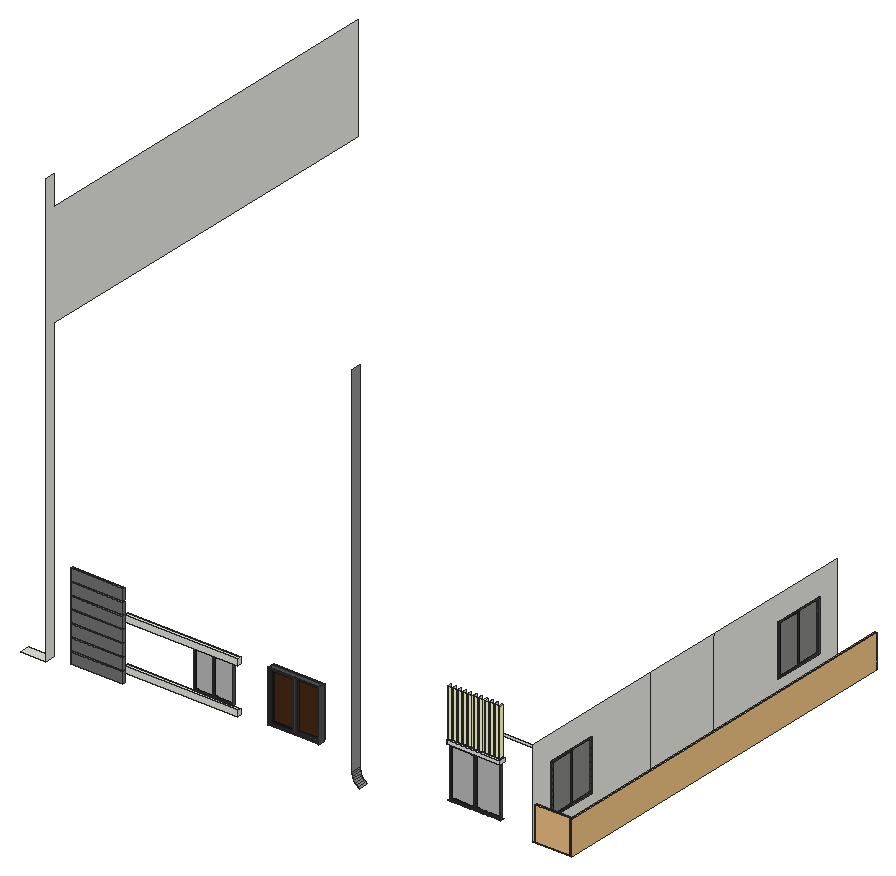
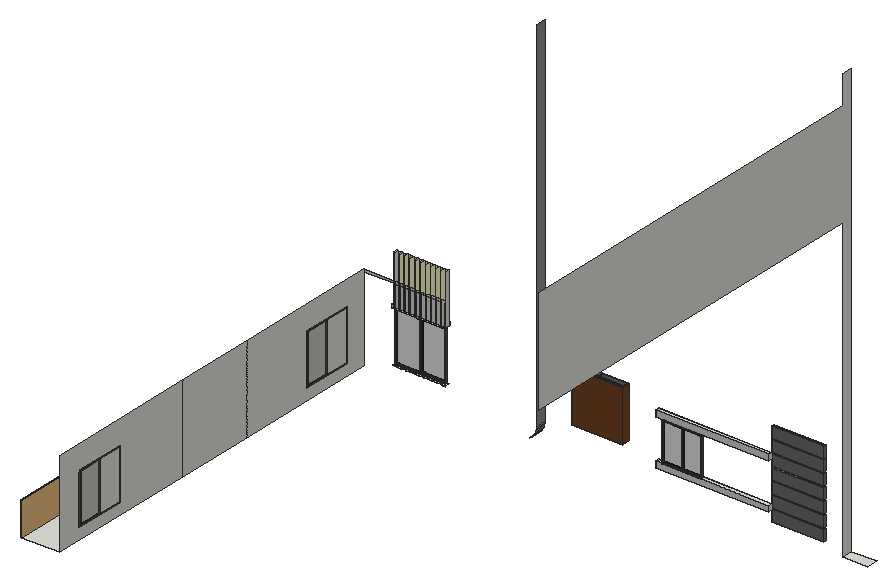
# SketchUp Ruby script. Lengths in inches.
U = 1.inch
M = Sketchup.active_model
def pt(a) = Geom::Point3d.new(a.map { |v| v * U })
def face(e, loops, mat)
  f = e.add_face(loops[0].map { |a| pt(a) })
  loops[1..].each { |l| e.add_face(l.map { |a| pt(a) }).erase! }
  f.material = f.back_material = mat if mat
  f
end
# faces: each face lists its corners as indices into pts; further lists are holes
def faces(e, pts, list, mat = nil) = list.each { |f| face(e, (f[0].is_a?(Array) ? f : [f]).map { |l| l.map { |i| pts[i] } }, mat) }
# xy, xz, yz: faces in a plane at the given z, y or x. An outline is a flat list of corners, or four numbers for a rectangle; further outlines are holes
def ring(l) = l.size == 4 ? [[l[0], l[1]], [l[2], l[1]], [l[2], l[3]], [l[0], l[3]]] : l.each_slice(2).to_a
def flat(e, list, mat, &to3) = list.each { |f| face(e, (f[0].is_a?(Array) ? f : [f]).map { |l| ring(l).map { |u, v| to3.(u, v) } }, mat) }
def xy(e, z, list, mat = nil) = flat(e, list, mat) { |x, y| [x, y, z] }
def xz(e, y, list, mat = nil) = flat(e, list, mat) { |x, z| [x, y, z] }
def yz(e, x, list, mat = nil) = flat(e, list, mat) { |y, z| [x, y, z] }
def lines(e, pts, list) = list.each { |a, b| e.add_line(pt(pts[a]), pt(pts[b])) }
# prism: a flat outline (further loops are holes) pulled along v
def prism(e, loops, v, mat = nil)
  f = face(e, loops, mat); d = Geom::Vector3d.new(v.map { |x| x * U })
  f.pushpull(f.normal.samedirection?(d) ? d.length : -d.length)
end
def box(e, o, s, mat = nil) = prism(e, [[o, [o[0] + s[0], o[1], o[2]], [o[0] + s[0], o[1] + s[1], o[2]], [o[0], o[1] + s[1], o[2]]]], [0, 0, s[2]], mat)
def at(x, y, z, deg = 0) = Geom::Transformation.translation(pt([x, y, z])) * Geom::Transformation.rotation(ORIGIN, Z_AXIS, deg.degrees)
def axes(o, x, y, z) = Geom::Transformation.new([*x, 0, *y, 0, *z, 0, *pt(o).to_a, 1])
def part(name) = M.definitions.add(name)
# library, detail: a bought-in or finely detailed component or shape, given as its bounding box
def library(name, o, s) = part(name).tap { |d| box(d.entities, o, s) }
def detail(e, o, s) = box(e.add_group.entities, o, s)
def put(e, d, t, mat = nil) = e.add_instance(d, t).tap { |i| i.material = mat if mat }
def group(e, t, mat = nil) = e.add_group.tap { |g| g.transformation = t; g.material = mat if mat }.entities
root = M.entities
M.materials.add("Glass_Tinted_Gray").color = [0, 0, 0]
M.materials["Glass_Tinted_Gray"].alpha = 0.125
M.materials.add("[0135_DarkGray]").color = [81, 81, 81]
M.materials.add("[Color E01]").color = [255, 255, 204]
M.materials.add("[Color M04]").color = [142, 142, 142]
M.materials.add("[Color M05]").color = [114, 114, 114]
M.materials.add("[Mirror 02]").color = [229, 229, 229]
M.materials.add("[Terrazzo Light Blue]").color = [196, 214, 227]
M.materials.add("[Wood Veneer 01]").color = [120, 70, 37]
c1 = library("Wagner Glass Railing",[9.08,102.375,1.53],[2.51,145.5,42.05])
c2 = part("Group\#9")
box(c2.entities,[0,-2.75,0],[65.625,2.75,13.9375])
c3 = part("PENTEK_RP Fineline 50S_Sliding_DoorCase_E1")
box(c3.entities,[0,0,0],[1.51,3.66,99.27],"[0135_DarkGray]")
c4 = part("PENTEK_RP Fineline 50S_SlidingDooe_Case_E2")
box(c4.entities,[0,0,0],[96.25,3.66,1.51],"[0135_DarkGray]")
c5 = part("pentek_RP Fineline 50S_SlidingDoor_Case")
put(c5.entities,c3,at(97.76,0,0))
put(c5.entities,c4,at(1.51,0,0))
put(c5.entities,c3,at(0,0,0))
put(c5.entities,c4,at(1.51,0,97.76))
c6 = part("PENTEK_RP Fineline 50S_SlidingDoor_GlazingBead_2")
box(c6.entities,[0,0,0],[0.56,0.59,94.39],"[0135_DarkGray]")
c7 = part("PENTEK_RP Fineline 50S_SlidingDoor_Glass")
box(c7.entities,[0,0,0],[46.58,0.16,94.39],"Glass_Tinted_Gray")
c8 = part("PENTEK_RP Fineline 50S_SlidingDoor_GlazingBead")
box(c8.entities,[0,0,0],[45.47,0.59,0.56],"[0135_DarkGray]")
c9 = part("PENTEK_RP Fineline 50S_SlidingDoor_Leaf_E1")
xy(c9.entities,0,[[0,0,0.93,1.97],[0.93,1.57,1.49,1.97]],"[0135_DarkGray]")
xy(c9.entities,96.25,[[0,0,0.93,0,0.93,1.57,1.49,1.57,1.49,1.97,0,1.97]],"[0135_DarkGray]")
xz(c9.entities,0,[[0,0,0.93,96.25]],"[0135_DarkGray]")
xz(c9.entities,1.57,[[0.93,0,1.49,95.32],[0.93,95.32,1.49,96.25]],"[0135_DarkGray]")
xz(c9.entities,1.97,[[0,0,1.49,96.25]],"[0135_DarkGray]")
yz(c9.entities,0,[[0,0,1.97,96.25]],"[0135_DarkGray]")
yz(c9.entities,0.93,[[0,0,1.57,0.93],[0,0.93,1.57,95.32],[0,95.32,1.57,96.25]],"[0135_DarkGray]")
yz(c9.entities,1.49,[[1.57,0,1.97,95.32],[1.57,95.32,1.97,96.25]],"[0135_DarkGray]")
c10 = part("PENTEK_RP Fineline 50S_SlidingDoor_Leaf_E2")
xy(c10.entities,0,[[0,0,0,1.57,0.56,1.57,0.56,1.97,46.02,1.97,46.02,1.57,46.58,1.57,46.58,0]],"[0135_DarkGray]")
xy(c10.entities,0.93,[[0,0,46.58,1.57]],"[0135_DarkGray]")
xy(c10.entities,1.49,[[0.56,1.57,46.02,1.97]],"[0135_DarkGray]")
xz(c10.entities,0,[[0,0,46.58,0.93]],"[0135_DarkGray]")
xz(c10.entities,1.57,[[0,0,0.56,0.93],[46.02,0,46.58,0.93],[0.56,0.93,46.02,1.49]],"[0135_DarkGray]")
xz(c10.entities,1.97,[[0.56,0,46.02,1.49]],"[0135_DarkGray]")
yz(c10.entities,0,[[0,0,1.57,0.93]],"[0135_DarkGray]")
yz(c10.entities,0.56,[[1.57,0,1.97,0.93],[1.57,0.93,1.97,1.49]],"[0135_DarkGray]")
yz(c10.entities,46.02,[[1.57,0,1.97,0.93],[1.57,0.93,1.97,1.49]],"[0135_DarkGray]")
yz(c10.entities,46.58,[[0,0,1.57,0.93]],"[0135_DarkGray]")
c11 = part("PENTEK_RP Fineline S_SlidingDoor_Leaf1")
put(c11.entities,c6,at(0.93,0,0.93))
put(c11.entities,c6,at(46.96,0,0.93))
put(c11.entities,c7,at(1.49,1.42,0.93))
put(c11.entities,c8,at(1.49,0,0.93))
put(c11.entities,c7,at(1.49,0.59,0.93),"[Terrazzo Light Blue]")
put(c11.entities,c9,at(0,0,0))
put(c11.entities,c9,axes([48.44,0,0],[-1,0,0],[0,1,0],[0,0,1]))
put(c11.entities,c10,axes([0.93,0,96.25],[1,0,0],[0,1,0],[0,0,-1]))
put(c11.entities,c10,at(0.93,0,0))
put(c11.entities,c8,at(1.49,0,94.77))
c12 = part("PENTEK_RP Fineline 50S_SlidingDoor_Leaf2")
put(c12.entities,c7,at(1.49,1.42,0.93))
put(c12.entities,c8,at(1.49,0,94.77))
put(c12.entities,c6,at(46.96,0,0.93))
put(c12.entities,c7,at(1.49,0.59,0.93),"[Mirror 02]")
put(c12.entities,c6,at(0.93,0,0.93))
put(c12.entities,c9,at(0,0,0))
put(c12.entities,c9,axes([48.44,0,0],[-1,0,0],[0,1,0],[0,0,1]))
put(c12.entities,c8,at(1.49,0,0.93))
put(c12.entities,c10,axes([0.93,0,96.25],[1,0,0],[0,1,0],[0,0,-1]))
put(c12.entities,c10,at(0.93,0,0))
c13 = part("PENTEK - Slimmest Steel Sliding Door / Window\#1")
put(c13.entities,c5,at(0,-1.88,-0.09))
put(c13.entities,c11,at(1.51,-2.27,1.42))
put(c13.entities,c12,at(49.32,-0.3,1.42))
c14 = part("Group\#10")
box(c14.entities,[-76.71,-4.875,-2.4375],[142.83,4.875,7.6875])
xy(root,7.25,[[7.375,49.27,39.25,62.39]])
xy(root,10.57,[[643.25,62.39,690.1875,542.39]])
xy(root,23.9,[[540.26,57.14,545.19,62.39],[545.88,57.14,550.82,62.39],[551.38,57.14,556.32,62.39],[557.13,57.14,562.07,62.39],[562.82,57.14,567.76,62.39],
  [568.44,57.14,573.38,62.39],[574.07,57.14,579.01,62.39],[579.51,57.14,584.44,62.39],[585.32,57.14,590.26,62.39],[590.94,57.14,595.88,62.39],
  [596.88,57.14,601.82,62.39],[602.25,57.14,607.1875,62.39]])
xy(root,34.3125,[[318.6,50.27,382.47,59.77]],"[Wood Veneer 01]")
xy(root,88.25,[[540.59,54.54,608.4,62.39]])
xy(root,90.0625,[[540.39,57.14,540.59,62.39],[540.59,57.14,545.76,62.39],[546.71,57.14,552.08,62.39],[553.03,57.14,558.4,62.39],[559.28,57.14,564.65,62.39],
  [565.65,57.14,571.03,62.39],[572.84,57.14,578.21,62.39],[579.65,57.14,585.03,62.39],[586.71,57.14,592.09,62.39],[592.73,57.14,598.11,62.39],
  [599.11,57.14,606.05,62.39]])
xy(root,93.1875,[[540.59,54.54,608.4,54.54,608.4,62.39,606.05,62.39,606.05,57.14,599.11,57.14,599.11,62.39,598.11,62.39,598.11,57.14,592.73,57.14,592.73,62.39,592.09,62.39,592.09,57.14,586.71,57.14,586.71,62.39,585.03,62.39,585.03,57.14,579.65,57.14,579.65,62.39,578.21,62.39,578.21,57.14,572.84,57.14,572.84,62.39,571.03,62.39,571.03,57.14,565.65,57.14,565.65,62.39,564.65,62.39,564.65,57.14,559.28,57.14,559.28,62.39,558.4,62.39,558.4,57.14,553.03,57.14,553.03,62.39,552.08,62.39,552.08,57.14,546.71,57.14,546.71,62.39,545.76,62.39,545.76,57.14,540.59,57.14]])
xy(root,98.1875,[[318.6,50.27,382.47,59.77]],"[Wood Veneer 01]")
xz(root,54.54,[[540.59,88.25,608.4,93.1875]])
xz(root,57.14,[[540.59,90.0625,545.76,93.1875],[546.71,90.0625,546.91,93.1875],[546.91,90.0625,552.08,93.1875],[553.03,90.0625,553.23,93.1875],[553.23,90.0625,558.4,93.1875],
  [559.28,90.0625,559.48,93.1875],[559.48,90.0625,564.65,93.1875],[565.65,90.0625,565.85,93.1875],[565.85,90.0625,571.03,93.1875],[572.84,90.0625,573.04,93.1875],
  [573.04,90.0625,578.21,93.1875],[579.65,90.0625,579.85,93.1875],[579.85,90.0625,585.03,93.1875],[586.71,90.0625,586.92,93.1875],[586.92,90.0625,592.09,93.1875],
  [592.73,90.0625,592.9375,93.1875],[592.9375,90.0625,598.11,93.1875],[599.11,90.0625,599.3125,93.1875],[604.48,90.0625,606.05,93.1875]])
xz(root,57.14,[[540.39,90.0625,540.59,90.0625,540.59,93.1875,545.76,93.1875,545.76,152.27,540.39,152.27],[599.3125,90.0625,604.48,90.0625,604.48,93.1875,606.05,93.1875,606.05,152.27,604.48,152.27,604.48,93.1875,599.3125,93.1875],[546.71,93.1875,552.08,152.27],[553.03,93.1875,558.4,152.27],[559.28,93.1875,564.65,152.27],
  [565.65,93.1875,571.03,152.27],[572.84,93.1875,578.21,152.27],[579.65,93.1875,585.03,152.27],[586.71,93.1875,592.09,152.27],[592.73,93.1875,598.11,152.27],
  [599.11,93.1875,604.48,152.27]],"[Color E01]")
xz(root,59.77,[[318.6,34.3125,382.47,98.1875]],"[Wood Veneer 01]")
xz(root,62.39,[[540.39,90.0625,541.21,116.82],[541.21,90.0625,545.76,90.0625,545.76,120,540.39,120,540.39,116.82,541.21,116.82],[546.71,90.0625,552.08,116.82],[553.03,90.0625,558.4,116.82],[559.28,90.0625,564.65,116.82],
  [565.65,90.0625,571.03,116.82],[572.84,90.0625,578.21,116.82],[579.65,90.0625,585.03,116.82],[586.71,90.0625,592.09,116.82],[592.73,90.0625,598.11,116.82],
  [599.11,90.0625,604.48,116.82],[604.48,90.0625,606.05,116.82],[545.76,93.1875,546.27,93.1875,546.27,116.82,546.71,116.82,546.71,120,545.76,120],[546.27,93.1875,546.71,116.82],[552.08,93.1875,553.03,116.82],
  [558.4,93.1875,559.28,116.82],[564.65,93.1875,565.65,116.82],[571.03,93.1875,572.84,116.82],[578.21,93.1875,579.65,116.82],[585.03,93.1875,586.71,116.82],
  [592.09,93.1875,592.73,116.82],[598.11,93.1875,599.11,116.82],[539.4375,116.82,540.39,120],[546.71,116.82,552.08,120],[552.08,116.82,553.03,120],
  [553.03,116.82,558.4,120],[558.4,116.82,559.28,120],[559.28,116.82,564.65,116.82,564.65,119.69,561.41,119.69,561.41,120,559.28,120],[564.65,116.82,565.65,119.69],[565.65,116.82,571.03,119.69],
  [571.03,116.82,572.84,119.69],[572.84,116.82,578.21,119.69],[578.21,116.82,579.65,119.69],[579.65,116.82,585.03,119.69],[585.03,116.82,586.71,119.69],
  [586.71,116.82,592.09,119.69],[592.09,116.82,592.73,119.69],[592.73,116.82,598.11,119.69],[598.11,116.82,599.11,119.69],[599.11,116.82,604.48,119.69],
  [604.48,116.82,606.05,119.69],[606.05,116.82,643.25,119.69]])
yz(root,39.25,[[49.27,7.25,49.27,552.6875,62.39,552.6875,62.39,516,542.39,516,542.39,384,62.39,384,62.39,7.25]])
yz(root,318.6,[[50.27,34.3125,59.77,98.1875]],"[Wood Veneer 01]")
yz(root,382.47,[[50.27,34.3125,59.77,98.1875]],"[Wood Veneer 01]")
yz(root,425.1875,[[50.27,18.35,62.39,472.24]],"[Color M04]")
yz(root,540.39,[[57.14,90.0625,62.39,152.27]])
yz(root,540.59,[[54.54,88.25,54.54,93.1875,57.14,93.1875,57.14,90.0625,62.39,90.0625,62.39,88.25]])
yz(root,545.76,[[57.14,90.0625,62.39,93.1875]])
yz(root,545.76,[[57.14,93.1875,62.39,152.27]],"[Color E01]")
yz(root,546.71,[[57.14,90.0625,62.39,93.1875],[57.14,93.1875,62.39,152.27]])
yz(root,552.08,[[57.14,90.0625,62.39,93.1875]])
yz(root,552.08,[[57.14,93.1875,62.39,152.27]],"[Color E01]")
yz(root,553.03,[[57.14,90.0625,62.39,93.1875],[57.14,93.1875,62.39,152.27]])
yz(root,558.4,[[57.14,90.0625,62.39,93.1875]])
yz(root,558.4,[[57.14,93.1875,62.39,152.27]],"[Color E01]")
yz(root,559.28,[[57.14,90.0625,62.39,93.1875],[57.14,93.1875,62.39,152.27]])
yz(root,564.65,[[57.14,90.0625,62.39,93.1875]])
yz(root,564.65,[[57.14,93.1875,62.39,152.27]],"[Color E01]")
yz(root,565.65,[[57.14,90.0625,62.39,93.1875],[57.14,93.1875,62.39,152.27]])
yz(root,571.03,[[57.14,90.0625,62.39,93.1875]])
yz(root,571.03,[[57.14,93.1875,62.39,152.27]],"[Color E01]")
yz(root,572.84,[[57.14,90.0625,62.39,93.1875],[57.14,93.1875,62.39,152.27]])
yz(root,578.21,[[57.14,90.0625,62.39,93.1875]])
yz(root,578.21,[[57.14,93.1875,62.39,152.27]],"[Color E01]")
yz(root,579.65,[[57.14,90.0625,62.39,93.1875],[57.14,93.1875,62.39,152.27]])
yz(root,585.03,[[57.14,90.0625,62.39,93.1875]])
yz(root,585.03,[[57.14,93.1875,62.39,152.27]],"[Color E01]")
yz(root,586.71,[[57.14,90.0625,62.39,93.1875],[57.14,93.1875,62.39,152.27]])
yz(root,592.09,[[57.14,90.0625,62.39,93.1875]])
yz(root,592.09,[[57.14,93.1875,62.39,152.27]],"[Color E01]")
yz(root,592.73,[[57.14,90.0625,62.39,93.1875],[57.14,93.1875,62.39,152.27]])
yz(root,598.11,[[57.14,90.0625,62.39,93.1875]])
yz(root,598.11,[[57.14,93.1875,62.39,152.27]],"[Color E01]")
yz(root,599.11,[[57.14,90.0625,62.39,93.1875],[57.14,93.1875,62.39,152.27]])
yz(root,604.48,[[57.14,90.0625,62.39,152.27]])
yz(root,606.05,[[57.14,90.0625,62.39,93.1875]])
yz(root,606.05,[[57.14,93.1875,62.39,152.27]],"[Color E01]")
yz(root,608.4,[[54.54,88.25,62.39,93.1875]])
yz(root,643.25,[[62.39,10.57,247.78,119.69],[247.78,10.57,348.35,119.69],[348.35,10.57,542.39,119.69]])
p = [[432.36,50.27,3.79],[434.36,50.27,2.46],[434.36,62.39,2.46],[432.36,62.39,3.79],[430.5625,50.27,5.375],[430.5625,62.39,5.375],
  [428.98,50.27,7.18],[428.98,62.39,7.18],[427.65,50.27,9.17],[427.65,62.39,9.17],[426.58,50.27,11.33],[426.58,62.39,11.33],
  [425.8125,50.27,13.6],[425.8125,62.39,13.6],[425.34,50.27,15.95],[425.34,62.39,15.95],[425.1875,50.27,18.35],[425.1875,62.39,18.35],
  [540.97,62.39,22.71],[545.19,62.39,22.71],[546.27,62.39,88.63],[541.21,62.39,88.63],[541.21,62.39,90.0625],[540.97,62.39,21.58],
  [546.27,62.39,93.1875]]
faces(root,p,[[0,1,2,3],[4,0,3,5],[6,4,5,7],[8,6,7,9],[10,8,9,11],[12,10,11,13],[14,12,13,15],[16,14,15,17]],"[Color M04]")
lines(root,p,[[18,19],[20,21],[21,22],[23,18],[24,20]])
put(root,c1,axes([612.93,74.81,9.03],[0,-1,0],[0.3167,0,0],[0,0,1]))
put(root,c1,axes([681.11,-275.34,9.03],[1,0,0],[0,3.29897,0],[0,0,1]))
put(root,c2,at(67.04,57.77,12.0625),"[Color M05]")
put(root,c13,axes([542.36,58.36,23.96],[0.6478,0,0],[0,0.6478,0],[0,0,0.6478]))
put(root,c14,at(209.375,61.89,26.66))
put(root,c13,axes([644.07,447.53,25.54],[0,0.6478,0],[-0.6478,0,0],[0,0,0.6478]))
put(root,c13,axes([644.07,89.22,25.54],[0,0.6478,0],[-0.6478,0,0],[0,0,0.6478]))
put(root,c2,at(67.04,57.77,27.75),"[Color M05]")
put(root,c13,axes([217.18,61.75,32.55],[0.5,0,0],[0,0.5,0],[0,0,0.5]))
put(root,c13,axes([319.34,53.68,34.375],[0.6481,0,0],[0,1.8178,0],[0,0,0.6534]))
put(root,c2,at(67.04,57.77,43.4375),"[Color M05]")
put(root,c2,at(67.04,57.77,59.125),"[Color M05]")
put(root,c2,at(67.04,57.77,74.8125),"[Color M05]")
put(root,c14,at(209.375,61.89,84.47))
put(root,c2,at(67.04,57.77,90.5),"[Color M05]")
put(root,c2,at(67.04,57.77,106.1875),"[Color M05]")
